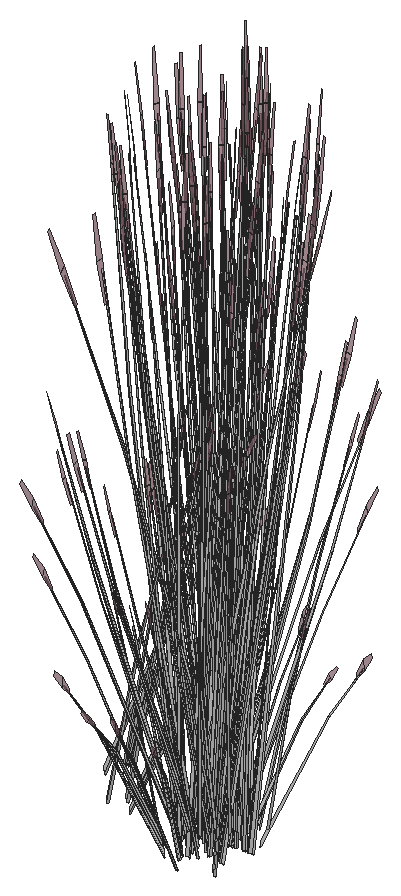
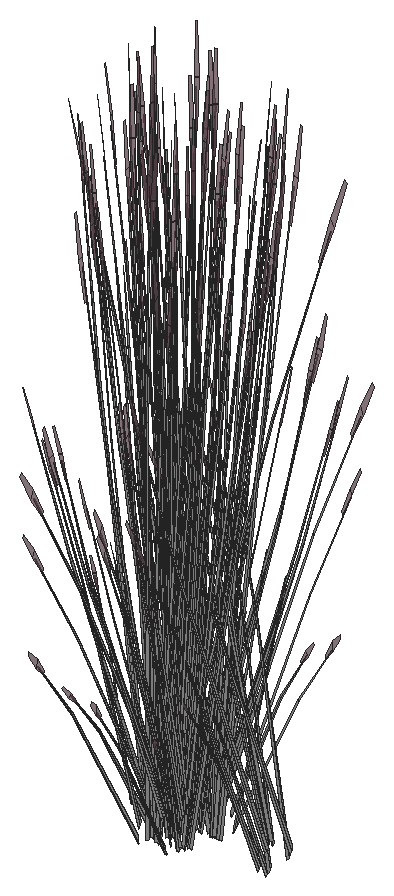
# SketchUp Ruby script. Lengths in inches.
U = 1.inch
M = Sketchup.active_model
def pt(a) = Geom::Point3d.new(a.map { |v| v * U })
def face(e, loops, mat)
  f = e.add_face(loops[0].map { |a| pt(a) })
  loops[1..].each { |l| e.add_face(l.map { |a| pt(a) }).erase! }
  f.material = f.back_material = mat if mat
  f
end
# faces: each face lists its corners as indices into pts; further lists are holes
def faces(e, pts, list, mat = nil) = list.each { |f| face(e, (f[0].is_a?(Array) ? f : [f]).map { |l| l.map { |i| pts[i] } }, mat) }
# xy, xz, yz: faces in a plane at the given z, y or x. An outline is a flat list of corners, or four numbers for a rectangle; further outlines are holes
def ring(l) = l.size == 4 ? [[l[0], l[1]], [l[2], l[1]], [l[2], l[3]], [l[0], l[3]]] : l.each_slice(2).to_a
def flat(e, list, mat, &to3) = list.each { |f| face(e, (f[0].is_a?(Array) ? f : [f]).map { |l| ring(l).map { |u, v| to3.(u, v) } }, mat) }
def xy(e, z, list, mat = nil) = flat(e, list, mat) { |x, y| [x, y, z] }
def xz(e, y, list, mat = nil) = flat(e, list, mat) { |x, z| [x, y, z] }
def yz(e, x, list, mat = nil) = flat(e, list, mat) { |y, z| [x, y, z] }
def lines(e, pts, list) = list.each { |a, b| e.add_line(pt(pts[a]), pt(pts[b])) }
# prism: a flat outline (further loops are holes) pulled along v
def prism(e, loops, v, mat = nil)
  f = face(e, loops, mat); d = Geom::Vector3d.new(v.map { |x| x * U })
  f.pushpull(f.normal.samedirection?(d) ? d.length : -d.length)
end
def box(e, o, s, mat = nil) = prism(e, [[o, [o[0] + s[0], o[1], o[2]], [o[0] + s[0], o[1] + s[1], o[2]], [o[0], o[1] + s[1], o[2]]]], [0, 0, s[2]], mat)
def at(x, y, z, deg = 0) = Geom::Transformation.translation(pt([x, y, z])) * Geom::Transformation.rotation(ORIGIN, Z_AXIS, deg.degrees)
def axes(o, x, y, z) = Geom::Transformation.new([*x, 0, *y, 0, *z, 0, *pt(o).to_a, 1])
def part(name) = M.definitions.add(name)
# library, detail: a bought-in or finely detailed component or shape, given as its bounding box
def library(name, o, s) = part(name).tap { |d| box(d.entities, o, s) }
def detail(e, o, s) = box(e.add_group.entities, o, s)
def put(e, d, t, mat = nil) = e.add_instance(d, t).tap { |i| i.material = mat if mat }
def group(e, t, mat = nil) = e.add_group.tap { |g| g.transformation = t; g.material = mat if mat }.entities
root = M.entities
M.materials.add("LightPink_Translucent").color = [144, 107, 117]
M.materials["LightPink_Translucent"].alpha = 0.75
M.materials.add("[_0053_Ivory_]").color = [200, 200, 200]
c1 = part("blade")
p = [[2.15,0.21,22],[0,0.17,0],[0.09,0.45,0],[2.18,0.31,22],[2.29,0.31,22],[0.38,0.45,0],
  [2.48,0.24,33],[2.49,0.24,33],[2.48,0.22,33]]
faces(c1.entities,p,[[0,1,2,3],[4,5,2,3],[6,3,4,7],[8,0,3,6]])
c2 = part("seeds")
p = [[0.3,-0.1,1.38],[-0.01,-0.03,1.59],[-0.01,-0.03,0.03],[0.14,-0.07,-0.07],[0.29,-0.03,3],[0.15,0.01,3.11]]
faces(c2.entities,p,[[0,1,2,3],[1,0,4,5]],"LightPink_Translucent")
c3 = part("blade with seeds")
put(c3.entities,c1,at(0,0,0))
put(c3.entities,c2,axes([2.4,0.25,30.99],[1.5799,-0.05474,1.17369],[-0.12525,1.92788,0.29478],[-0.07173,-0.02425,1.56792]))
put(root,c3,axes([468.92,100.3125,131.33],[-0.59932,0.14948,-0.51099],[-0.10484,-0.56611,-0.3958],[-0.16097,-0.16223,0.97773]),"[_0053_Ivory_]")
put(root,c3,axes([468.4,104.48,128.67],[-0.56842,-0.31443,-0.49651],[0.33976,-0.56381,0],[-0.12946,-0.07161,1.57504]),"[_0053_Ivory_]")
put(root,c3,axes([468.15,99.8,128.15],[-0.05883,0.08284,1.76342],[-0.59454,0.17861,-0.26939],[-0.14363,-0.16248,0.30037]),"[_0053_Ivory_]")
put(root,c3,axes([468.74,104.86,129.03],[-0.37973,0.63014,0],[-0.6353,-0.35142,-0.51607],[-0.14469,-0.08004,1.63711]),"[_0053_Ivory_]")
put(root,c3,axes([461.2,103.5625,131.33],[0.16454,-0.57202,-0.51099],[0.56413,0.19607,-0.3958],[0.22713,-0.05245,0.97773]),"[_0053_Ivory_]")
put(root,c3,axes([462.62,103.93,129.42],[-0.37526,0.10382,1.1486],[0.17664,-0.42906,0.84392],[0.19907,0.02936,0.25299]),"[_0053_Ivory_]")
put(root,c3,axes([461.41,102.0625,129.24],[-0.21697,-0.01863,1.43002],[-0.22228,-0.49966,-0.30754],[0.26655,-0.14135,0.61141]),"[_0053_Ivory_]")
put(root,c3,axes([468.05,105.77,129.24],[0.19166,-0.0992,1.43002],[0.4732,0.29912,-0.30754],[-0.14084,0.25882,0.61141]),"[_0053_Ivory_]")
put(root,c3,axes([461.55,103.82,131.18],[0.50475,0.17543,-0.35414],[-0.14722,0.5118,0.4572],[0.20322,-0.04693,0.87481]),"[_0053_Ivory_]")
put(root,c3,axes([467.78,100.11,128.78],[-0.1752,0.51349,-0.03893],[-0.53924,-0.15795,-0.17649],[-0.08187,-0.08399,0.58215]),"[_0053_Ivory_]")
put(root,c3,axes([460.58,104.93,131.63],[0.60713,0.01514,-0.71045],[-0.04078,0.63759,0.08574],[0.25721,0.06729,1.00501]),"[_0053_Ivory_]")
put(root,c3,axes([468.58,99.47,129.24],[-0.03678,0.20572,1.43002],[-0.53767,0.17221,-0.30754],[-0.12568,-0.26589,0.61141]),"[_0053_Ivory_]")
put(root,c3,axes([461.81,103.72,128.64],[-0.39118,0.07547,1.41583],[-0.06226,-0.6007,0.08104],[0.27398,-0.09092,0.80566]),"[_0053_Ivory_]")
put(root,c3,axes([468.76,100,130.53],[0.13883,0.2019,1.71376],[-0.64153,0.16998,0.13857],[-0.14499,-0.31697,0.73262]),"[_0053_Ivory_]")
put(root,c3,axes([469.94,103.37,129.32],[-0.61322,0.4175,-0.29095],[-0.40778,-0.58992,-0.50002],[-0.1513,-0.05991,1.59708]),"[_0053_Ivory_]")
put(root,c3,axes([462.23,103.33,128.15],[-0.03174,-0.09547,1.76342],[0.22015,-0.55846,-0.26939],[0.22208,-0.00803,0.30037]),"[_0053_Ivory_]")
put(root,c3,axes([460.18,103.19,130.53],[-0.25192,0.01424,1.71376],[0.16712,-0.61729,0.13857],[0.35901,0.03818,0.73262]),"[_0053_Ivory_]")
put(root,c3,axes([468.98,99.89,131.18],[-0.0938,-0.50652,-0.35414],[0.53623,-0.13375,0.4572],[-0.14403,-0.14515,0.87481]),"[_0053_Ivory_]")
put(root,c3,axes([467.49,102.46,129.03],[-0.75945,0,0],[0,-0.70283,-0.51607],[0,-0.16007,1.63711]),"[_0053_Ivory_]")
put(root,c3,axes([468.55,104.24,128.68],[-0.14267,-0.54795,-0.30978],[0.56663,-0.1556,0.30978],[-0.11423,-0.06319,1.38974]),"[_0053_Ivory_]")
put(root,c3,axes([468.25,104.82,131.18],[-0.41095,0.33109,-0.35414],[-0.38901,-0.37805,0.4572],[-0.05919,0.19208,0.87481]),"[_0053_Ivory_]")
put(root,c3,axes([461.1,103.77,131.63],[0.53369,-0.27773,-0.71045],[0.29743,0.5717,0.08574],[0.25786,-0.06494,1.00501]),"[_0053_Ivory_]")
put(root,c3,axes([470.35,103.82,128.71],[-0.40909,0.47266,-0.62353],[-0.50819,-0.4286,-0.16365],[-0.16393,0.11791,1.37633]),"[_0053_Ivory_]")
put(root,c3,axes([468.08,102.27,128.98],[-0.56493,0.5287,0.30756],[-0.56528,-0.52313,-0.36492],[-0.01973,-0.15014,1.64885]),"[_0053_Ivory_]")
put(root,c3,axes([470.4,103.73,129.98],[0.52485,0.25358,1.51261],[-0.51417,0.54629,0.59816],[-0.23031,-0.32378,1.26806]),"[_0053_Ivory_]")
put(root,c3,axes([468.4,99.14,129.42],[0.31682,0.21887,1.1486],[-0.4614,0.13157,0.84392],[-0.09872,-0.16821,0.25299]),"[_0053_Ivory_]")
put(root,c3,axes([470.63,103.56,129.12],[-0.59306,-0.50614,-0.25192],[0.49904,-0.56836,0.5513],[-0.1597,0.05921,1.68216]),"[_0053_Ivory_]")
put(root,c3,axes([469.55,103.07,128.86],[-0.36485,-0.52782,-0.44739],[0.55265,-0.37168,0.21531],[-0.11807,-0.06531,1.43643]),"[_0053_Ivory_]")
put(root,c3,axes([468.52,104.47,131.99],[-0.0158,0.58168,-0.7886],[-0.66548,-0.03907,0.09517],[-0.07023,0.24643,1.11556]),"[_0053_Ivory_]")
put(root,c3,axes([461.92,104.62,129.24],[-0.14627,-0.15466,1.43002],[0.19032,-0.51164,-0.30754],[0.29594,0.06931,0.61141]),"[_0053_Ivory_]")
put(root,c3,axes([468.51,106.1,129.42],[-0.01572,-0.37392,1.1486],[0.39276,0.26669,0.84392],[-0.07724,0.17822,0.25299]),"[_0053_Ivory_]")
put(root,c3,axes([470.33,103.45,128.86],[-0.65953,0.03882,-0.44739],[-0.05964,-0.64439,0.21531],[-0.11807,0.06531,1.43643]),"[_0053_Ivory_]")
put(root,c3,axes([469.07,104.53,129.13],[0.56842,0.31443,0.49651],[-0.33976,0.56381,0],[-0.12946,-0.07161,1.57504]),"[_0053_Ivory_]")
put(root,c3,axes([468.3,105.29,130.02],[0.01334,-0.32463,1.54345],[0.60018,0.17147,0.21329],[-0.052,0.34598,0.72882]),"[_0053_Ivory_]")
put(root,c3,axes([469.61,103.375,129.09],[0.16098,-0.74515,-0.23429],[0.76326,0.12989,0.51271],[-0.13337,-0.1029,1.5644]),"[_0053_Ivory_]")
put(root,c3,axes([469.88,103.55,129.27],[-0.11717,0.56122,0.1448],[-0.57245,-0.09742,-0.41347],[-0.10418,-0.05763,1.26744]),"[_0053_Ivory_]")
put(root,c3,axes([471.02,105.11,128.67],[-0.56842,0.31443,-0.49651],[-0.33976,-0.56381,0],[-0.12946,0.07161,1.57504]),"[_0053_Ivory_]")
put(root,c3,axes([467.66,101.98,128.67],[0,-0.62885,-0.49651],[0.67951,0,0],[0,-0.14322,1.57504]),"[_0053_Ivory_]")
put(root,c3,axes([467.95,102.57,129.13],[0,0.62885,0.49651],[-0.67951,0,0],[0,-0.14322,1.57504]),"[_0053_Ivory_]")
put(root,c3,axes([471.0625,104.95,128.85],[-0.37499,-0.63235,-0.05142],[0.6353,-0.35142,0.51607],[-0.15655,0.0602,1.6363]),"[_0053_Ivory_]")
put(root,c3,axes([468.66,104.66,131.66],[0.43478,0.42253,-0.5672],[-0.45929,0.37004,-0.43934],[-0.06615,0.21468,1.08528]),"[_0053_Ivory_]")
put(root,c3,axes([470.89,104.87,128.68],[-0.56663,-0.1556,-0.30978],[0.14267,-0.54795,0.30978],[-0.11423,0.06319,1.38974]),"[_0053_Ivory_]")
put(root,c3,axes([469.43,102.71,129.32],[-0.68399,-0.30005,-0.29095],[0.32934,-0.63331,-0.50002],[-0.0215,-0.15549,1.59708]),"[_0053_Ivory_]")
put(root,c3,axes([471.22,102.52,129.5],[-0.01659,-0.59209,1.41272],[0.75089,0.15348,0.59816],[-0.1776,0.32398,1.3335]),"[_0053_Ivory_]")
put(root,c3,axes([468.18,105.29,129.48],[0.55175,-0.11136,0.06507],[0.12684,0.44864,-0.86304],[-0.03498,0.22711,0.7736]),"[_0053_Ivory_]")
put(root,c3,axes([470.79,103.28,129.32],[0.07077,0.71755,-0.29095],[-0.73712,0.04339,-0.50002],[-0.1298,0.09558,1.59708]),"[_0053_Ivory_]")
put(root,c3,axes([469.13,102.07,128.75],[-0.24943,-0.64486,-0.69835],[0.71849,-0.23224,-0.18329],[-0.02757,-0.21836,1.54149]),"[_0053_Ivory_]")
put(root,c3,axes([470.25,100.05,131.33],[-0.59704,-0.15764,-0.51099],[0.20464,-0.54049,-0.3958],[-0.05475,-0.21761,0.97773]),"[_0053_Ivory_]")
put(root,c3,axes([469.15,104.05,130.53],[-0.01487,-0.24136,1.71376],[0.64429,0.16012,0.13857],[-0.03985,0.34396,0.73262]),"[_0053_Ivory_]")
put(root,c3,axes([467.95,102,128.68],[0.42396,-0.39235,-0.30978],[0.42396,0.39235,0.30978],[0,-0.12637,1.38974]),"[_0053_Ivory_]")
put(root,c3,axes([469.86,99.46,128.78],[-0.4197,0.36076,-0.03893],[-0.38456,-0.39511,-0.17649],[-0.02707,-0.11196,0.58215]),"[_0053_Ivory_]")
put(root,c3,axes([469.7,103.02,129.01],[0.76764,0.13249,0.45755],[-0.15622,0.74829,0.17955],[-0.11218,-0.07226,1.58856]),"[_0053_Ivory_]")
put(root,c3,axes([469.5,102.88,129.37],[-0.29468,0.56664,0.44739],[-0.61229,-0.27271,-0.21531],[0,-0.13062,1.43643]),"[_0053_Ivory_]")
put(root,c3,axes([470.47,100.15,131.63],[-0.28988,-0.51132,-0.71045],[0.59671,-0.28496,0.08574],[-0.06778,-0.24706,1.00501]),"[_0053_Ivory_]")
put(root,c3,axes([469.28,104.21,129.13],[0.65264,-0.16691,0.17642],[0.16115,0.62115,0.35086],[-0.05821,-0.0905,1.60407]),"[_0053_Ivory_]")
put(root,c3,axes([470.12,104.31,128.85],[-0.61229,-0.28233,0],[0.29468,-0.58663,0],[0,0,1.62707]),"[_0053_Ivory_]")
put(root,c3,axes([471.54,105.02,129.03],[0.37973,0.63014,0],[-0.6353,0.35142,-0.51607],[-0.14469,0.08004,1.63711]),"[_0053_Ivory_]")
put(root,c3,axes([471.23,104.25,129.13],[0.17545,-0.62497,0.17642],[0.64204,0.17686,0.35086],[-0.11091,0.00304,1.60407]),"[_0053_Ivory_]")
put(root,c3,axes([470.93,103.42,129.27],[0.44871,0.37783,0.1448],[-0.37428,0.42627,-0.41347],[-0.10418,0.05763,1.26744]),"[_0053_Ivory_]")
put(root,c3,axes([470.77,102.95,128.95],[-0.56493,-0.54126,-0.06131],[0.56528,-0.54159,0],[-0.01973,-0.0189,1.75571]),"[_0053_Ivory_]")
put(root,c3,axes([470.92,103.14,129.37],[0.65953,-0.03882,0.44739],[0.05964,0.64439,-0.21531],[-0.11807,0.06531,1.43643]),"[_0053_Ivory_]")
put(root,c3,axes([471.08,104.62,128.98],[0.76036,0.2044,0.30756],[-0.19023,0.7306,-0.36492],[-0.12585,0.09144,1.64885]),"[_0053_Ivory_]")
put(root,c3,axes([469.97,99.02,128.15],[-0.10187,0.02266,1.76342],[-0.56336,-0.25503,-0.26939],[0.00945,-0.21273,0.30037]),"[_0053_Ivory_]")
put(root,c3,axes([471.41,104.58,129.13],[0.56842,-0.31443,0.49651],[0.33976,0.56381,0],[-0.12946,0.07161,1.57504]),"[_0053_Ivory_]")
put(root,c3,axes([470.52,99.72,131.18],[0.1831,-0.48359,-0.35414],[0.53419,0.14105,0.4572],[-0.04898,-0.1947,0.87481]),"[_0053_Ivory_]")
put(root,c3,axes([469.63,102.33,129.01],[0.26406,0.70318,0.45755],[-0.7545,0.24452,0.17955],[0.00922,-0.12921,1.58856]),"[_0053_Ivory_]")
put(root,c3,axes([469.51,102.24,128.86],[0.29468,-0.56664,-0.44739],[0.61229,0.27271,0.21531],[0,-0.13062,1.43643]),"[_0053_Ivory_]")
put(root,c3,axes([470.26,104.07,128.86],[-0.19817,-0.54216,0],[0.56587,-0.18986,0],[0,0,1.54371]),"[_0053_Ivory_]")
put(root,c3,axes([469.54,105.21,128.15],[0.09829,-0.03422,1.76342],[0.59126,0.18834,-0.26939],[0.01729,0.21228,0.30037]),"[_0053_Ivory_]")
put(root,c3,axes([469.67,105.4,131.18],[-0.1831,0.48359,-0.35414],[-0.53419,-0.14105,0.4572],[0.04898,0.1947,0.87481]),"[_0053_Ivory_]")
put(root,c3,axes([471.0625,103,128.86],[-0.29468,0.56664,-0.44739],[-0.61229,-0.27271,0.21531],[0,0.13062,1.43643]),"[_0053_Ivory_]")
put(root,c3,axes([472.23,102.65,129.13],[-0.47719,-0.45806,0.17642],[0.48088,-0.44429,0.35086],[-0.0527,0.09355,1.60407]),"[_0053_Ivory_]")
put(root,c3,axes([470.58,102.39,128.86],[0,-0.72763,0],[0.75945,0,0],[0,0,1.79456]),"[_0053_Ivory_]")
put(root,c3,axes([469.87,102.52,129.09],[0.68433,0.30479,0.24065],[-0.32934,0.63331,0.50002],[0,-0.14599,1.60543]),"[_0053_Ivory_]")
put(root,c3,axes([470.96,102.68,128.95],[0,0.72727,-0.05637],[-0.75945,0,0],[0,0.02286,1.79368]),"[_0053_Ivory_]")
put(root,c3,axes([469.65,102.09,129.37],[-0.65953,0.03882,0.44739],[-0.05964,-0.64439,-0.21531],[0.11807,-0.06531,1.43643]),"[_0053_Ivory_]")
put(root,c3,axes([469.34,100.99,129.13],[-0.17545,0.62497,0.17642],[-0.64204,-0.17686,0.35086],[0.11091,-0.00304,1.60407]),"[_0053_Ivory_]")
put(root,c3,axes([470.6,104.08,128.94],[0.26406,0.72244,-0.06012],[-0.7545,0.25315,0],[0.00922,0.02523,1.72173]),"[_0053_Ivory_]")
put(root,c3,axes([469.03,100.22,129.03],[-0.37973,-0.63014,0],[0.6353,-0.35142,-0.51607],[0.14469,-0.08004,1.63711]),"[_0053_Ivory_]")
put(root,c3,axes([469.73,104.97,131.63],[0.28988,0.51132,-0.71045],[-0.59671,0.28496,0.08574],[0.06778,0.24706,1.00501]),"[_0053_Ivory_]")
put(root,c3,axes([472.78,103.14,128.85],[-0.75908,-0.00503,-0.04976],[0,-0.70283,0.49943],[-0.02386,0.16,1.58352]),"[_0053_Ivory_]")
put(root,c3,axes([471.29,101.02,129.13],[-0.65264,0.16691,0.17642],[-0.16115,-0.62115,0.35086],[0.05821,0.0905,1.60407]),"[_0053_Ivory_]")
put(root,c3,axes([470.62,98.69,129.42],[0.07791,0.3667,1.1486],[-0.43222,-0.2031,0.84392],[0.04651,-0.18776,0.25299]),"[_0053_Ivory_]")
put(root,c3,axes([470.22,101.93,129.01],[-0.50358,0.57069,0.45755],[-0.59827,-0.50377,0.17955],[0.1214,-0.05695,1.58856]),"[_0053_Ivory_]")
put(root,c3,axes([471.08,102.83,128.87],[0.42396,0.40619,0],[-0.42396,0.40619,0],[0,0,1.69266]),"[_0053_Ivory_]")
put(root,c3,axes([471.07,102.35,129.37],[0.29468,-0.56664,0.44739],[0.61229,0.27271,-0.21531],[0,0.13062,1.43643]),"[_0053_Ivory_]")
put(root,c3,axes([470.82,104.32,128.86],[0.61229,0.28233,0],[-0.29468,0.58663,0],[0,0,1.74954]),"[_0053_Ivory_]")
put(root,c3,axes([469.95,105.07,131.33],[0.59704,0.15764,-0.51099],[-0.20464,0.54049,-0.3958],[0.05475,0.21761,0.97773]),"[_0053_Ivory_]")
put(root,c3,axes([470.875,102.22,129.03],[-0.76764,-0.13249,0.49198],[0.15622,-0.74829,0.19306],[0.11218,0.07226,1.70813]),"[_0053_Ivory_]")
put(root,c3,axes([472.62,103.24,128.68],[-0.42396,0.39235,-0.30978],[-0.42396,-0.39235,0.30978],[0,0.12637,1.38974]),"[_0053_Ivory_]")
put(root,c3,axes([471.41,103.17,128.75],[0.2227,0.57576,-0.69212],[-0.64151,0.20736,-0.18165],[0.02462,0.19497,1.52773]),"[_0053_Ivory_]")
put(root,c3,axes([471.09,102.55,128.86],[0.67951,0,0],[0,0.65103,0],[0,0,1.78407]),"[_0053_Ivory_]")
put(root,c3,axes([470.44,101.83,129.37],[-0.36485,-0.52782,0.44739],[0.55265,-0.37168,-0.21531],[0.11807,0.06531,1.43643]),"[_0053_Ivory_]")
put(root,c3,axes([469.78,101.96,129.32],[-0.07077,-0.71755,-0.29095],[0.73712,-0.04339,-0.50002],[0.1298,-0.09558,1.59708]),"[_0053_Ivory_]")
put(root,c3,axes([471.33,102.48,129.27],[0.56587,-0.18339,0.1448],[0.19817,0.52368,-0.41347],[0,0.11525,1.26744]),"[_0053_Ivory_]")
put(root,c3,axes([471.54,100.46,131.33],[-0.43478,-0.42253,-0.51099],[0.45929,-0.37004,-0.3958],[0.06615,-0.21468,0.97773]),"[_0053_Ivory_]")
put(root,c3,axes([471.14,102.53,129.32],[0.68399,0.30005,-0.29095],[-0.32934,0.63331,-0.50002],[0.0215,0.15549,1.59708]),"[_0053_Ivory_]")
put(root,c3,axes([469.68,100.37,128.68],[0.56663,0.1556,-0.30978],[-0.14267,0.54795,0.30978],[0.11423,-0.06319,1.38974]),"[_0053_Ivory_]")
put(root,c3,axes([471.26,99.71,129.24],[-0.17264,0.12729,1.43002],[-0.51703,-0.22279,-0.30754],[0.09584,-0.27707,0.61141]),"[_0053_Ivory_]")
put(root,c3,axes([472.62,102.67,129.13],[0,-0.62885,0.49651],[0.67951,0,0],[0,0.14322,1.57504]),"[_0053_Ivory_]")
put(root,c3,axes([472.91,103.25,128.67],[0,0.62885,-0.49651],[-0.67951,0,0],[0,0.14322,1.57504]),"[_0053_Ivory_]")
put(root,c3,axes([469.55,100.12,128.67],[0.56842,-0.31443,-0.49651],[0.33976,0.56381,0],[0.12946,-0.07161,1.57504]),"[_0053_Ivory_]")
put(root,c3,axes([470.28,103.95,130.53],[-0.13883,-0.2019,1.71376],[0.64153,-0.16998,0.13857],[0.14499,0.31697,0.73262]),"[_0053_Ivory_]")
put(root,c3,axes([470.69,101.68,129.27],[0.11717,-0.56122,0.1448],[0.57245,0.09742,-0.41347],[0.10418,0.05763,1.26744]),"[_0053_Ivory_]")
put(root,c3,axes([471.5,100.71,129.13],[-0.56842,-0.31443,0.49651],[0.33976,-0.56381,0],[0.12946,0.07161,1.57504]),"[_0053_Ivory_]")
put(root,c3,axes([471.68,100.65,131.63],[0.0158,-0.58168,-0.71045],[0.66548,0.03907,0.08574],[0.07023,-0.24643,1.00501]),"[_0053_Ivory_]")
put(root,c3,axes([471,103.99,128.84],[0.63764,-0.21337,-0.19198],[0.22406,0.61462,0.00008],[0.07038,-0.02358,1.73897]),"[_0053_Ivory_]")
put(root,c3,axes([471.02,102.16,128.86],[0.36485,0.52782,-0.44739],[-0.55265,0.37168,0.21531],[0.11807,0.06531,1.43643]),"[_0053_Ivory_]")
put(root,c3,axes([471.95,100.3,131.18],[0.41095,-0.33109,-0.35414],[0.38901,0.37805,0.4572],[0.05919,-0.19208,0.87481]),"[_0053_Ivory_]")
put(root,c3,axes([472.05,104.56,129.42],[-0.34197,-0.18082,1.1486],[0.44156,-0.18372,0.84392],[0.1191,0.15563,0.25299]),"[_0053_Ivory_]")
put(root,c3,axes([470.83,104.36,129.24],[0.01072,-0.20846,1.43002],[0.51218,-0.23285,-0.30754],[0.15811,0.2495,0.61141]),"[_0053_Ivory_]")
put(root,c3,axes([470.22,101.41,128.71],[0.40909,-0.47266,-0.62353],[0.50819,0.4286,-0.16365],[0.16393,-0.11791,1.37633]),"[_0053_Ivory_]")
put(root,c3,axes([472.01,100.99,128.68],[0.14267,0.54795,-0.30978],[-0.56663,0.1556,0.30978],[0.11423,0.06319,1.38974]),"[_0053_Ivory_]")
put(root,c3,axes([473.08,102.78,129.03],[0.75945,0,0],[0,0.70283,-0.51607],[0,0.16007,1.63711]),"[_0053_Ivory_]")
put(root,c3,axes([470.63,101.87,129.32],[0.61322,-0.4175,-0.29095],[0.40778,0.58992,-0.50002],[0.1513,0.05991,1.59708]),"[_0053_Ivory_]")
put(root,c3,axes([472.1,105.38,129.32],[-0.38947,-0.01972,1.0506],[0.25721,-0.41888,0.58006],[0.15386,0.14882,0.8241]),"[_0053_Ivory_]")
put(root,c3,axes([470.93,100.36,130.53],[-0.11309,0.21615,1.71376],[-0.47441,-0.44731,0.13857],[0.21402,-0.27879,0.73262]),"[_0053_Ivory_]")
put(root,c3,axes([469.08,101.49,128.25],[-0.59782,0.25177,1.28929],[-0.19028,-0.72239,0.50096],[0.36709,0.01202,1.46642]),"[_0053_Ivory_]")
put(root,c3,axes([471.28,104.81,131.33],[0.59932,-0.14948,-0.51099],[0.10484,0.56611,-0.3958],[0.16097,0.16223,0.97773]),"[_0053_Ivory_]")
put(root,c3,axes([471.83,100.375,129.03],[0.37973,-0.63014,0],[0.6353,0.35142,-0.51607],[0.14469,0.08004,1.63711]),"[_0053_Ivory_]")
put(root,c3,axes([472.46,100.1,128.15],[-0.0909,-0.04954,1.76342],[-0.2335,-0.55347,-0.26939],[0.15752,-0.1502,0.30037]),"[_0053_Ivory_]")
put(root,c3,axes([472.17,100.76,128.67],[0.56842,0.31443,-0.49651],[-0.33976,0.56381,0],[0.12946,0.07161,1.57504]),"[_0053_Ivory_]")
put(root,c3,axes([472.14,105.23,128.15],[0.04425,-0.09079,1.76342],[0.55709,-0.26738,-0.26939],[0.16889,0.13839,0.30037]),"[_0053_Ivory_]")
put(root,c3,axes([472.44,101.43,131.33],[-0.15602,-0.5742,-0.51099],[0.59087,-0.10045,-0.3958],[0.16933,-0.15423,0.97773]),"[_0053_Ivory_]")
put(root,c3,axes([473.48,104.39,130.58],[-0.11624,-0.52862,-0.03492],[0.54943,-0.12153,-0.15832],[0.11473,0.03351,0.52218]),"[_0053_Ivory_]")
